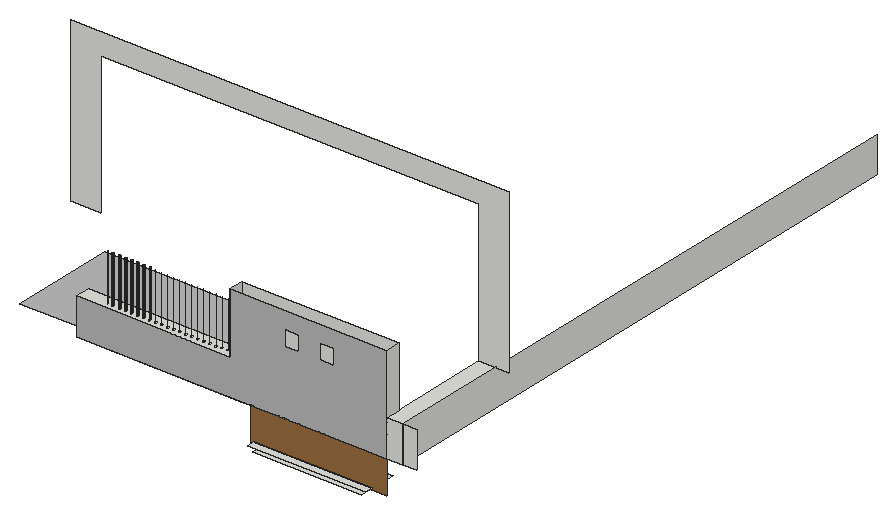
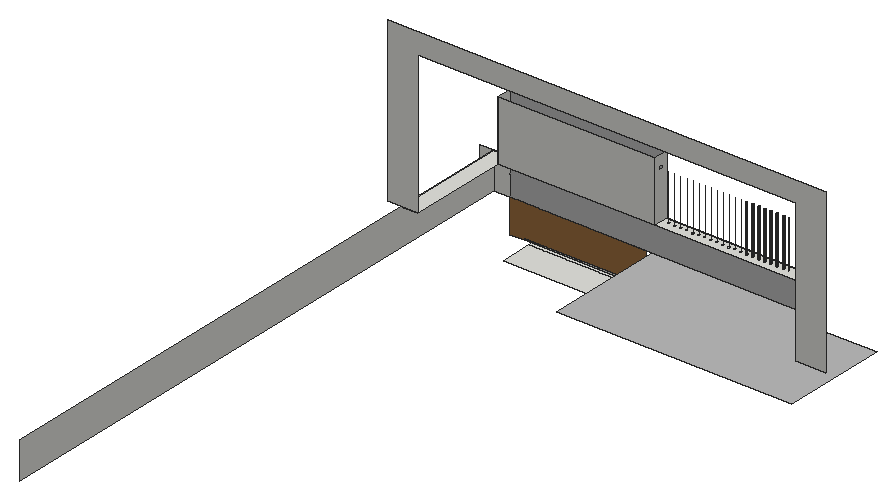
# SketchUp Ruby script. Lengths in inches.
U = 1.inch
M = Sketchup.active_model
def pt(a) = Geom::Point3d.new(a.map { |v| v * U })
def face(e, loops, mat)
  f = e.add_face(loops[0].map { |a| pt(a) })
  loops[1..].each { |l| e.add_face(l.map { |a| pt(a) }).erase! }
  f.material = f.back_material = mat if mat
  f
end
# faces: each face lists its corners as indices into pts; further lists are holes
def faces(e, pts, list, mat = nil) = list.each { |f| face(e, (f[0].is_a?(Array) ? f : [f]).map { |l| l.map { |i| pts[i] } }, mat) }
# xy, xz, yz: faces in a plane at the given z, y or x. An outline is a flat list of corners, or four numbers for a rectangle; further outlines are holes
def ring(l) = l.size == 4 ? [[l[0], l[1]], [l[2], l[1]], [l[2], l[3]], [l[0], l[3]]] : l.each_slice(2).to_a
def flat(e, list, mat, &to3) = list.each { |f| face(e, (f[0].is_a?(Array) ? f : [f]).map { |l| ring(l).map { |u, v| to3.(u, v) } }, mat) }
def xy(e, z, list, mat = nil) = flat(e, list, mat) { |x, y| [x, y, z] }
def xz(e, y, list, mat = nil) = flat(e, list, mat) { |x, z| [x, y, z] }
def yz(e, x, list, mat = nil) = flat(e, list, mat) { |y, z| [x, y, z] }
def lines(e, pts, list) = list.each { |a, b| e.add_line(pt(pts[a]), pt(pts[b])) }
# prism: a flat outline (further loops are holes) pulled along v
def prism(e, loops, v, mat = nil)
  f = face(e, loops, mat); d = Geom::Vector3d.new(v.map { |x| x * U })
  f.pushpull(f.normal.samedirection?(d) ? d.length : -d.length)
end
def box(e, o, s, mat = nil) = prism(e, [[o, [o[0] + s[0], o[1], o[2]], [o[0] + s[0], o[1] + s[1], o[2]], [o[0], o[1] + s[1], o[2]]]], [0, 0, s[2]], mat)
def at(x, y, z, deg = 0) = Geom::Transformation.translation(pt([x, y, z])) * Geom::Transformation.rotation(ORIGIN, Z_AXIS, deg.degrees)
def axes(o, x, y, z) = Geom::Transformation.new([*x, 0, *y, 0, *z, 0, *pt(o).to_a, 1])
def part(name) = M.definitions.add(name)
# library, detail: a bought-in or finely detailed component or shape, given as its bounding box
def library(name, o, s) = part(name).tap { |d| box(d.entities, o, s) }
def detail(e, o, s) = box(e.add_group.entities, o, s)
def put(e, d, t, mat = nil) = e.add_instance(d, t).tap { |i| i.material = mat if mat }
def group(e, t, mat = nil) = e.add_group.tap { |g| g.transformation = t; g.material = mat if mat }.entities
root = M.entities
M.materials.add("Generic").color = [155, 110, 63]
M.materials.add("Generic\#2").color = [186, 186, 186]
xy(root,951.29,[[543.83,116.625,654.26,124.5],[540.39,124.5,654.26,156.8125]])
xy(root,955.48,[[538.69,116.625,658.46,124.5]])
xy(root,987.75,[[359.25,124.5,359.25,138.74,290.4375,138.74,290.4375,246,528.75,246,528.75,124.5]],"Generic\#2")
xy(root,1024.625,[[483.23,129.75,483.02,129.78,482.82,129.86,482.66,129.99,482.53,130.16,482.45,130.36,482.42,130.57,482.45,130.78,482.53,130.97,482.66,131.14,482.82,131.27,483.02,131.35,483.23,131.38,483.44,131.35,483.64,131.27,483.81,131.14,483.93,130.97,484.02,130.78,484.04,130.57,484.02,130.36,483.93,130.16,483.81,129.99,483.64,129.86,483.44,129.78]])
xy(root,1024.6875,[[[359.25,124.5,514.86,139.4375],[501.61,129.75,501.4,129.78,501.2,129.86,501.03,129.99,500.9,130.16,500.82,130.36,500.79,130.57,500.82,130.78,500.9,130.97,501.03,131.14,501.2,131.27,501.4,131.35,501.61,131.38,501.82,131.35,502.01,131.27,502.18,131.14,502.31,130.97,502.39,130.78,502.42,130.57,502.39,130.36,502.31,130.16,502.18,129.99,502.01,129.86,501.82,129.78],[495.61,129.75,495.4,129.78,495.2,129.86,495.03,129.99,494.9,130.16,494.82,130.36,494.79,130.57,494.82,130.78,494.9,130.97,495.03,131.14,495.2,131.27,495.4,131.35,495.61,131.38,495.82,131.35,496.01,131.27,496.18,131.14,496.31,130.97,496.39,130.78,496.42,130.57,496.39,130.36,496.31,130.16,496.18,129.99,496.01,129.86,495.82,129.78],[489.61,129.75,489.4,129.78,489.2,129.86,489.03,129.99,488.9,130.16,488.82,130.36,488.79,130.57,488.82,130.78,488.9,130.97,489.03,131.14,489.2,131.27,489.4,131.35,489.61,131.38,489.82,131.35,490.01,131.27,490.18,131.14,490.31,130.97,490.39,130.78,490.42,130.57,490.39,130.36,490.31,130.16,490.18,129.99,490.01,129.86,489.82,129.78],[483.23,129.75,483.02,129.78,482.82,129.86,482.66,129.99,482.53,130.16,482.45,130.36,482.42,130.57,482.45,130.78,482.53,130.97,482.66,131.14,482.82,131.27,483.02,131.35,483.23,131.38,483.44,131.35,483.64,131.27,483.81,131.14,483.93,130.97,484.02,130.78,484.04,130.57,484.02,130.36,483.93,130.16,483.81,129.99,483.64,129.86,483.44,129.78],[477.17,129.75,476.96,129.78,476.76,129.86,476.59,129.99,476.46,130.16,476.38,130.36,476.36,130.57,476.38,130.78,476.46,130.97,476.59,131.14,476.76,131.27,476.96,131.35,477.17,131.38,477.38,131.35,477.57,131.27,477.74,131.14,477.87,130.97,477.95,130.78,477.98,130.57,477.95,130.36,477.87,130.16,477.74,129.99,477.57,129.86,477.38,129.78],[471.17,129.75,470.96,129.78,470.76,129.86,470.59,129.99,470.46,130.16,470.38,130.36,470.36,130.57,470.38,130.78,470.46,130.97,470.59,131.14,470.76,131.27,470.96,131.35,471.17,131.38,471.38,131.35,471.57,131.27,471.74,131.14,471.87,130.97,471.95,130.78,471.98,130.57,471.95,130.36,471.87,130.16,471.74,129.99,471.57,129.86,471.38,129.78],[464.79,129.75,464.58,129.78,464.39,129.86,464.22,129.99,464.09,130.16,464.01,130.36,463.98,130.57,464.01,130.78,464.09,130.97,464.22,131.14,464.39,131.27,464.58,131.35,464.79,131.38,465,131.35,465.2,131.27,465.37,131.14,465.5,130.97,465.58,130.78,465.61,130.57,465.58,130.36,465.5,130.16,465.37,129.99,465.2,129.86,465,129.78],[458.54,129.75,458.33,129.78,458.14,129.86,457.97,129.99,457.84,130.16,457.76,130.36,457.73,130.57,457.76,130.78,457.84,130.97,457.97,131.14,458.14,131.27,458.33,131.35,458.54,131.38,458.75,131.35,458.95,131.27,459.12,131.14,459.25,130.97,459.33,130.78,459.36,130.57,459.33,130.36,459.25,130.16,459.12,129.99,458.95,129.86,458.75,129.78],[452.61,129.75,452.4,129.78,452.2,129.86,452.03,129.99,451.9,130.16,451.82,130.36,451.79,130.57,451.82,130.78,451.9,130.97,452.03,131.14,452.2,131.27,452.4,131.35,452.61,131.38,452.82,131.35,453.01,131.27,453.18,131.14,453.31,130.97,453.39,130.78,453.42,130.57,453.39,130.36,453.31,130.16,453.18,129.99,453.01,129.86,452.82,129.78],[446.36,129.75,446.15,129.78,445.95,129.86,445.78,129.99,445.65,130.16,445.57,130.36,445.54,130.57,445.57,130.78,445.65,130.97,445.78,131.14,445.95,131.27,446.15,131.35,446.36,131.38,446.57,131.35,446.76,131.27,446.93,131.14,447.06,130.97,447.14,130.78,447.17,130.57,447.14,130.36,447.06,130.16,446.93,129.99,446.76,129.86,446.57,129.78],[440.36,129.75,440.15,129.78,439.95,129.86,439.78,129.99,439.65,130.16,439.57,130.36,439.54,130.57,439.57,130.78,439.65,130.97,439.78,131.14,439.95,131.27,440.15,131.35,440.36,131.38,440.57,131.35,440.76,131.27,440.93,131.14,441.06,130.97,441.14,130.78,441.17,130.57,441.14,130.36,441.06,130.16,440.93,129.99,440.76,129.86,440.57,129.78],[434.23,129.75,434.02,129.78,433.82,129.86,433.66,129.99,433.53,130.16,433.45,130.36,433.42,130.57,433.45,130.78,433.53,130.97,433.66,131.14,433.82,131.27,434.02,131.35,434.23,131.38,434.44,131.35,434.64,131.27,434.81,131.14,434.93,130.97,435.02,130.78,435.04,130.57,435.02,130.36,434.93,130.16,434.81,129.99,434.64,129.86,434.44,129.78],[428.17,129.75,427.96,129.78,427.76,129.86,427.59,129.99,427.46,130.16,427.38,130.36,427.36,130.57,427.38,130.78,427.46,130.97,427.59,131.14,427.76,131.27,427.96,131.35,428.17,131.38,428.38,131.35,428.57,131.27,428.74,131.14,428.87,130.97,428.95,130.78,428.98,130.57,428.95,130.36,428.87,130.16,428.74,129.99,428.57,129.86,428.38,129.78],[421.98,129.75,421.77,129.78,421.57,129.86,421.41,129.99,421.28,130.16,421.2,130.36,421.17,130.57,421.2,130.78,421.28,130.97,421.41,131.14,421.57,131.27,421.77,131.35,421.98,131.38,422.19,131.35,422.39,131.27,422.56,131.14,422.68,130.97,422.77,130.78,422.79,130.57,422.77,130.36,422.68,130.16,422.56,129.99,422.39,129.86,422.19,129.78],[415.86,129.75,415.65,129.78,415.45,129.86,415.28,129.99,415.15,130.16,415.07,130.36,415.04,130.57,415.07,130.78,415.15,130.97,415.28,131.14,415.45,131.27,415.65,131.35,415.86,131.38,416.07,131.35,416.26,131.27,416.43,131.14,416.56,130.97,416.64,130.78,416.67,130.57,416.64,130.36,416.56,130.16,416.43,129.99,416.26,129.86,416.07,129.78],[409.73,129.75,409.52,129.78,409.32,129.86,409.16,129.99,409.03,130.16,408.95,130.36,408.92,130.57,408.95,130.78,409.03,130.97,409.16,131.14,409.32,131.27,409.52,131.35,409.73,131.38,409.94,131.35,410.14,131.27,410.31,131.14,410.43,130.97,410.52,130.78,410.54,130.57,410.52,130.36,410.43,130.16,410.31,129.99,410.14,129.86,409.94,129.78],[403.61,129.75,403.4,129.78,403.2,129.86,403.03,129.99,402.9,130.16,402.82,130.36,402.79,130.57,402.82,130.78,402.9,130.97,403.03,131.14,403.2,131.27,403.4,131.35,403.61,131.38,403.82,131.35,404.01,131.27,404.18,131.14,404.31,130.97,404.39,130.78,404.42,130.57,404.39,130.36,404.31,130.16,404.18,129.99,404.01,129.86,403.82,129.78],[397.54,129.75,397.33,129.78,397.14,129.86,396.97,129.99,396.84,130.16,396.76,130.36,396.73,130.57,396.76,130.78,396.84,130.97,396.97,131.14,397.14,131.27,397.33,131.35,397.54,131.38,397.75,131.35,397.95,131.27,398.12,131.14,398.25,130.97,398.33,130.78,398.36,130.57,398.33,130.36,398.25,130.16,398.12,129.99,397.95,129.86,397.75,129.78],[391.23,129.75,391.02,129.78,390.82,129.86,390.66,129.99,390.53,130.16,390.45,130.36,390.42,130.57,390.45,130.78,390.53,130.97,390.66,131.14,390.82,131.27,391.02,131.35,391.23,131.38,391.44,131.35,391.64,131.27,391.81,131.14,391.93,130.97,392.02,130.78,392.04,130.57,392.02,130.36,391.93,130.16,391.81,129.99,391.64,129.86,391.44,129.78],[385.23,129.75,385.02,129.78,384.82,129.86,384.66,129.99,384.53,130.16,384.45,130.36,384.42,130.57,384.45,130.78,384.53,130.97,384.66,131.14,384.82,131.27,385.02,131.35,385.23,131.38,385.44,131.35,385.64,131.27,385.81,131.14,385.93,130.97,386.02,130.78,386.04,130.57,386.02,130.36,385.93,130.16,385.81,129.99,385.64,129.86,385.44,129.78],[378.98,129.75,378.77,129.78,378.57,129.86,378.41,129.99,378.28,130.16,378.2,130.36,378.17,130.57,378.2,130.78,378.28,130.97,378.41,131.14,378.57,131.27,378.77,131.35,378.98,131.38,379.19,131.35,379.39,131.27,379.56,131.14,379.68,130.97,379.77,130.78,379.79,130.57,379.77,130.36,379.68,130.16,379.56,129.99,379.39,129.86,379.19,129.78],[372.73,129.75,372.52,129.78,372.32,129.86,372.16,129.99,372.03,130.16,371.95,130.36,371.92,130.57,371.95,130.78,372.03,130.97,372.16,131.14,372.32,131.27,372.52,131.35,372.73,131.38,372.94,131.35,373.14,131.27,373.31,131.14,373.43,130.97,373.52,130.78,373.54,130.57,373.52,130.36,373.43,130.16,373.31,129.99,373.14,129.86,372.94,129.78],[366.79,129.75,366.58,129.78,366.39,129.86,366.22,129.99,366.09,130.16,366.01,130.36,365.98,130.57,366.01,130.78,366.09,130.97,366.22,131.14,366.39,131.27,366.58,131.35,366.79,131.38,367,131.35,367.2,131.27,367.37,131.14,367.5,130.97,367.58,130.78,367.61,130.57,367.58,130.36,367.5,130.16,367.37,129.99,367.2,129.86,367,129.78],[360.79,129.75,360.58,129.78,360.39,129.86,360.22,129.99,360.09,130.16,360.01,130.36,359.98,130.57,360.01,130.78,360.09,130.97,360.22,131.14,360.39,131.27,360.58,131.35,360.79,131.38,361,131.35,361.2,131.27,361.37,131.14,361.5,130.97,361.58,130.78,361.61,130.57,361.58,130.36,361.5,130.16,361.37,129.99,361.2,129.86,361,129.78],[507.61,129.75,507.4,129.78,507.2,129.86,507.03,129.99,506.9,130.16,506.82,130.36,506.79,130.57,506.82,130.78,506.9,130.97,507.03,131.14,507.2,131.27,507.4,131.35,507.61,131.38,507.82,131.35,508.01,131.27,508.18,131.14,508.31,130.97,508.39,130.78,508.42,130.57,508.39,130.36,508.31,130.16,508.18,129.99,508.01,129.86,507.82,129.78]],[673.48,124.5,690.4375,241.25],[391.23,129.75,391.02,129.78,390.82,129.86,390.66,129.99,390.53,130.16,390.45,130.36,390.42,130.57,390.45,130.78,390.53,130.97,390.66,131.14,390.82,131.27,391.02,131.35,391.23,131.38,391.44,131.35,391.64,131.27,391.81,131.14,391.93,130.97,392.02,130.78,392.04,130.57,392.02,130.36,391.93,130.16,391.81,129.99,391.64,129.86,391.44,129.78],[397.54,129.75,397.33,129.78,397.14,129.86,396.97,129.99,396.84,130.16,396.76,130.36,396.73,130.57,396.76,130.78,396.84,130.97,396.97,131.14,397.14,131.27,397.33,131.35,397.54,131.38,397.75,131.35,397.95,131.27,398.12,131.14,398.25,130.97,398.33,130.78,398.36,130.57,398.33,130.36,398.25,130.16,398.12,129.99,397.95,129.86,397.75,129.78],[403.61,129.75,403.4,129.78,403.2,129.86,403.03,129.99,402.9,130.16,402.82,130.36,402.79,130.57,402.82,130.78,402.9,130.97,403.03,131.14,403.2,131.27,403.4,131.35,403.61,131.38,403.82,131.35,404.01,131.27,404.18,131.14,404.31,130.97,404.39,130.78,404.42,130.57,404.39,130.36,404.31,130.16,404.18,129.99,404.01,129.86,403.82,129.78],
  [409.73,129.75,409.52,129.78,409.32,129.86,409.16,129.99,409.03,130.16,408.95,130.36,408.92,130.57,408.95,130.78,409.03,130.97,409.16,131.14,409.32,131.27,409.52,131.35,409.73,131.38,409.94,131.35,410.14,131.27,410.31,131.14,410.43,130.97,410.52,130.78,410.54,130.57,410.52,130.36,410.43,130.16,410.31,129.99,410.14,129.86,409.94,129.78],[415.86,129.75,415.65,129.78,415.45,129.86,415.28,129.99,415.15,130.16,415.07,130.36,415.04,130.57,415.07,130.78,415.15,130.97,415.28,131.14,415.45,131.27,415.65,131.35,415.86,131.38,416.07,131.35,416.26,131.27,416.43,131.14,416.56,130.97,416.64,130.78,416.67,130.57,416.64,130.36,416.56,130.16,416.43,129.99,416.26,129.86,416.07,129.78],[421.98,129.75,421.77,129.78,421.57,129.86,421.41,129.99,421.28,130.16,421.2,130.36,421.17,130.57,421.2,130.78,421.28,130.97,421.41,131.14,421.57,131.27,421.77,131.35,421.98,131.38,422.19,131.35,422.39,131.27,422.56,131.14,422.68,130.97,422.77,130.78,422.79,130.57,422.77,130.36,422.68,130.16,422.56,129.99,422.39,129.86,422.19,129.78],[428.17,129.75,427.96,129.78,427.76,129.86,427.59,129.99,427.46,130.16,427.38,130.36,427.36,130.57,427.38,130.78,427.46,130.97,427.59,131.14,427.76,131.27,427.96,131.35,428.17,131.38,428.38,131.35,428.57,131.27,428.74,131.14,428.87,130.97,428.95,130.78,428.98,130.57,428.95,130.36,428.87,130.16,428.74,129.99,428.57,129.86,428.38,129.78],[434.23,129.75,434.02,129.78,433.82,129.86,433.66,129.99,433.53,130.16,433.45,130.36,433.42,130.57,433.45,130.78,433.53,130.97,433.66,131.14,433.82,131.27,434.02,131.35,434.23,131.38,434.44,131.35,434.64,131.27,434.81,131.14,434.93,130.97,435.02,130.78,435.04,130.57,435.02,130.36,434.93,130.16,434.81,129.99,434.64,129.86,434.44,129.78],
  [440.36,129.75,440.15,129.78,439.95,129.86,439.78,129.99,439.65,130.16,439.57,130.36,439.54,130.57,439.57,130.78,439.65,130.97,439.78,131.14,439.95,131.27,440.15,131.35,440.36,131.38,440.57,131.35,440.76,131.27,440.93,131.14,441.06,130.97,441.14,130.78,441.17,130.57,441.14,130.36,441.06,130.16,440.93,129.99,440.76,129.86,440.57,129.78],[446.36,129.75,446.15,129.78,445.95,129.86,445.78,129.99,445.65,130.16,445.57,130.36,445.54,130.57,445.57,130.78,445.65,130.97,445.78,131.14,445.95,131.27,446.15,131.35,446.36,131.38,446.57,131.35,446.76,131.27,446.93,131.14,447.06,130.97,447.14,130.78,447.17,130.57,447.14,130.36,447.06,130.16,446.93,129.99,446.76,129.86,446.57,129.78],[452.61,129.75,452.4,129.78,452.2,129.86,452.03,129.99,451.9,130.16,451.82,130.36,451.79,130.57,451.82,130.78,451.9,130.97,452.03,131.14,452.2,131.27,452.4,131.35,452.61,131.38,452.82,131.35,453.01,131.27,453.18,131.14,453.31,130.97,453.39,130.78,453.42,130.57,453.39,130.36,453.31,130.16,453.18,129.99,453.01,129.86,452.82,129.78],[458.54,129.75,458.33,129.78,458.14,129.86,457.97,129.99,457.84,130.16,457.76,130.36,457.73,130.57,457.76,130.78,457.84,130.97,457.97,131.14,458.14,131.27,458.33,131.35,458.54,131.38,458.75,131.35,458.95,131.27,459.12,131.14,459.25,130.97,459.33,130.78,459.36,130.57,459.33,130.36,459.25,130.16,459.12,129.99,458.95,129.86,458.75,129.78],[464.79,129.75,464.58,129.78,464.39,129.86,464.22,129.99,464.09,130.16,464.01,130.36,463.98,130.57,464.01,130.78,464.09,130.97,464.22,131.14,464.39,131.27,464.58,131.35,464.79,131.38,465,131.35,465.2,131.27,465.37,131.14,465.5,130.97,465.58,130.78,465.61,130.57,465.58,130.36,465.5,130.16,465.37,129.99,465.2,129.86,465,129.78],
  [471.17,129.75,470.96,129.78,470.76,129.86,470.59,129.99,470.46,130.16,470.38,130.36,470.36,130.57,470.38,130.78,470.46,130.97,470.59,131.14,470.76,131.27,470.96,131.35,471.17,131.38,471.38,131.35,471.57,131.27,471.74,131.14,471.87,130.97,471.95,130.78,471.98,130.57,471.95,130.36,471.87,130.16,471.74,129.99,471.57,129.86,471.38,129.78],[477.17,129.75,476.96,129.78,476.76,129.86,476.59,129.99,476.46,130.16,476.38,130.36,476.36,130.57,476.38,130.78,476.46,130.97,476.59,131.14,476.76,131.27,476.96,131.35,477.17,131.38,477.38,131.35,477.57,131.27,477.74,131.14,477.87,130.97,477.95,130.78,477.98,130.57,477.95,130.36,477.87,130.16,477.74,129.99,477.57,129.86,477.38,129.78],[483.23,129.75,483.02,129.78,482.82,129.86,482.66,129.99,482.53,130.16,482.45,130.36,482.42,130.57,482.45,130.78,482.53,130.97,482.66,131.14,482.82,131.27,483.02,131.35,483.23,131.38,483.44,131.35,483.64,131.27,483.81,131.14,483.93,130.97,484.02,130.78,484.04,130.57,484.02,130.36,483.93,130.16,483.81,129.99,483.64,129.86,483.44,129.78],[489.61,129.75,489.4,129.78,489.2,129.86,489.03,129.99,488.9,130.16,488.82,130.36,488.79,130.57,488.82,130.78,488.9,130.97,489.03,131.14,489.2,131.27,489.4,131.35,489.61,131.38,489.82,131.35,490.01,131.27,490.18,131.14,490.31,130.97,490.39,130.78,490.42,130.57,490.39,130.36,490.31,130.16,490.18,129.99,490.01,129.86,489.82,129.78],[495.61,129.75,495.4,129.78,495.2,129.86,495.03,129.99,494.9,130.16,494.82,130.36,494.79,130.57,494.82,130.78,494.9,130.97,495.03,131.14,495.2,131.27,495.4,131.35,495.61,131.38,495.82,131.35,496.01,131.27,496.18,131.14,496.31,130.97,496.39,130.78,496.42,130.57,496.39,130.36,496.31,130.16,496.18,129.99,496.01,129.86,495.82,129.78],
  [501.61,129.75,501.4,129.78,501.2,129.86,501.03,129.99,500.9,130.16,500.82,130.36,500.79,130.57,500.82,130.78,500.9,130.97,501.03,131.14,501.2,131.27,501.4,131.35,501.61,131.38,501.82,131.35,502.01,131.27,502.18,131.14,502.31,130.97,502.39,130.78,502.42,130.57,502.39,130.36,502.31,130.16,502.18,129.99,502.01,129.86,501.82,129.78],[507.61,129.75,507.4,129.78,507.2,129.86,507.03,129.99,506.9,130.16,506.82,130.36,506.79,130.57,506.82,130.78,506.9,130.97,507.03,131.14,507.2,131.27,507.4,131.35,507.61,131.38,507.82,131.35,508.01,131.27,508.18,131.14,508.31,130.97,508.39,130.78,508.42,130.57,508.39,130.36,508.31,130.16,508.18,129.99,508.01,129.86,507.82,129.78]])
xz(root,124.5,[[538.69,954,658.46,955.48],[673.48,987.75,690.4375,1024.6875],[690.4375,987.75,703.6875,1024.6875]])
xz(root,124.5,[[535.75,954,538.69,954,538.69,955.48,658.46,955.48,658.46,954,673.48,954,673.48,987.75,535.75,987.75]],"Generic")
xz(root,124.5,[[[359.25,987.75,673.48,987.75,673.48,1085.75,514.86,1085.75,514.86,1024.6875,359.25,1024.6875],[570.42,1053.3125,584.1,1069],[605.79,1053.3125,619.48,1069]]],"Generic\#2")
xz(root,139.4375,[[514.86,1024.6875,673.48,1085.75]])
xz(root,241.25,[[259.3125,1024.6875,259.3125,1189.3125,703.6875,1189.3125,703.6875,1024.6875,673.48,1024.6875,673.48,1168.125,290.4375,1168.125,290.4375,1024.6875]])
yz(root,514.86,[[[124.5,1024.6875,139.4375,1085.75],[128.48,1072.38,133.48,1075.32]]])
yz(root,673.48,[[124.5,1024.6875,139.4375,1085.75]])
yz(root,690.4375,[[124.5,987.75,724.5,1024.6875]])
p = [[483.02,129.78,1024.6875],[482.82,129.86,1024.6875],[482.82,129.86,1024.625],[483.02,129.78,1024.625],[483.23,129.75,1024.6875],[483.23,129.75,1024.625],
  [483.44,129.78,1024.6875],[483.44,129.78,1024.625],[483.64,129.86,1024.6875],[483.64,129.86,1024.625],[482.66,129.99,1024.6875],[482.66,129.99,1024.625],
  [483.81,129.99,1024.6875],[483.81,129.99,1024.625],[482.53,130.16,1024.6875],[482.53,130.16,1024.625],[483.93,130.16,1024.6875],[483.93,130.16,1024.625],
  [482.45,130.36,1024.6875],[482.45,130.36,1024.625],[484.02,130.36,1024.6875],[484.02,130.36,1024.625],[482.42,130.57,1024.6875],[482.42,130.57,1024.625],
  [484.04,130.57,1024.6875],[484.04,130.57,1024.625],[482.45,130.78,1024.6875],[482.45,130.78,1024.625],[484.02,130.78,1024.6875],[484.02,130.78,1024.625],
  [482.53,130.97,1024.6875],[482.53,130.97,1024.625],[483.93,130.97,1024.6875],[483.93,130.97,1024.625],[482.66,131.14,1024.6875],[482.66,131.14,1024.625],
  [483.81,131.14,1024.6875],[483.81,131.14,1024.625],[482.82,131.27,1024.6875],[482.82,131.27,1024.625],[483.64,131.27,1024.6875],[483.64,131.27,1024.625],
  [483.02,131.35,1024.6875],[483.02,131.35,1024.625],[483.44,131.35,1024.6875],[483.44,131.35,1024.625],[483.23,131.38,1024.6875],[483.23,131.38,1024.625],
  [390.82,129.86,1024.6875],[391.02,129.78,1024.6875],[391.02,129.78,1072.38],[390.82,129.86,1072.38],[391.23,129.75,1024.6875],[391.23,129.75,1072.38],
  [391.44,129.78,1024.6875],[391.44,129.78,1072.38],[391.64,129.86,1024.6875],[391.64,129.86,1072.38],[397.14,129.86,1024.6875],[397.33,129.78,1024.6875],
  [397.33,129.78,1072.38],[397.14,129.86,1072.38],[397.54,129.75,1024.6875],[397.54,129.75,1072.38],[397.75,129.78,1024.6875],[397.75,129.78,1072.38],
  [397.95,129.86,1024.6875],[397.95,129.86,1072.38],[403.2,129.86,1024.6875],[403.4,129.78,1024.6875],[403.4,129.78,1072.38],[403.2,129.86,1072.38],
  [403.61,129.75,1024.6875],[403.61,129.75,1072.38],[403.82,129.78,1024.6875],[403.82,129.78,1072.38],[404.01,129.86,1024.6875],[404.01,129.86,1072.38],
  [409.32,129.86,1024.6875],[409.52,129.78,1024.6875],[409.52,129.78,1072.38],[409.32,129.86,1072.38],[409.73,129.75,1024.6875],[409.73,129.75,1072.38],
  [409.94,129.78,1024.6875],[409.94,129.78,1072.38],[410.14,129.86,1024.6875],[410.14,129.86,1072.38],[415.45,129.86,1024.6875],[415.65,129.78,1024.6875],
  [415.65,129.78,1072.38],[415.45,129.86,1072.38],[415.86,129.75,1024.6875],[415.86,129.75,1072.38],[416.07,129.78,1024.6875],[416.07,129.78,1072.38],
  [416.26,129.86,1024.6875],[416.26,129.86,1072.38],[421.57,129.86,1024.6875],[421.77,129.78,1024.6875],[421.77,129.78,1072.38],[421.57,129.86,1072.38],
  [421.98,129.75,1024.6875],[421.98,129.75,1072.38],[422.19,129.78,1024.6875],[422.19,129.78,1072.38],[422.39,129.86,1024.6875],[422.39,129.86,1072.38],
  [390.66,129.99,1024.6875],[390.66,129.99,1072.38],[391.81,129.99,1024.6875],[391.81,129.99,1072.38],[396.97,129.99,1024.6875],[396.97,129.99,1072.38],
  [398.12,129.99,1024.6875],[398.12,129.99,1072.38],[403.03,129.99,1024.6875],[403.03,129.99,1072.38],[404.18,129.99,1024.6875],[404.18,129.99,1072.38],
  [409.16,129.99,1024.6875],[409.16,129.99,1072.38],[410.31,129.99,1024.6875],[410.31,129.99,1072.38],[415.28,129.99,1024.6875],[415.28,129.99,1072.38],
  [416.43,129.99,1024.6875],[416.43,129.99,1072.38],[421.41,129.99,1024.6875],[421.41,129.99,1072.38],[422.56,129.99,1024.6875],[422.56,129.99,1072.38],
  [428.57,129.86,1024.6875],[428.74,129.99,1024.6875],[428.74,129.99,1072.38],[428.57,129.86,1072.38],[390.53,130.16,1024.6875],[390.53,130.16,1072.38],
  [391.93,130.16,1024.6875],[391.93,130.16,1072.38],[396.84,130.16,1024.6875],[396.84,130.16,1072.38],[398.25,130.16,1024.6875],[398.25,130.16,1072.38],
  [402.9,130.16,1024.6875],[402.9,130.16,1072.38],[404.31,130.16,1024.6875],[404.31,130.16,1072.38],[409.03,130.16,1024.6875],[409.03,130.16,1072.38],
  [410.43,130.16,1024.6875],[410.43,130.16,1072.38],[415.15,130.16,1024.6875],[415.15,130.16,1072.38],[416.56,130.16,1024.6875],[416.56,130.16,1072.38],
  [421.28,130.16,1024.6875],[421.28,130.16,1072.38],[422.68,130.16,1024.6875],[422.68,130.16,1072.38],[428.87,130.16,1024.6875],[428.87,130.16,1072.38],
  [390.45,130.36,1024.6875],[390.45,130.36,1072.38],[392.02,130.36,1024.6875],[392.02,130.36,1072.38],[396.76,130.36,1024.6875],[396.76,130.36,1072.38],
  [398.33,130.36,1024.6875],[398.33,130.36,1072.38],[402.82,130.36,1024.6875],[402.82,130.36,1072.38],[404.39,130.36,1024.6875],[404.39,130.36,1072.38],
  [408.95,130.36,1024.6875],[408.95,130.36,1072.38],[410.52,130.36,1024.6875],[410.52,130.36,1072.38],[415.07,130.36,1024.6875],[415.07,130.36,1072.38],
  [416.64,130.36,1024.6875],[416.64,130.36,1072.38],[421.2,130.36,1024.6875],[421.2,130.36,1072.38],[422.77,130.36,1024.6875],[422.77,130.36,1072.38],
  [428.95,130.36,1024.6875],[428.95,130.36,1072.38],[390.42,130.57,1024.6875],[390.42,130.57,1072.38],[392.04,130.57,1024.6875],[392.04,130.57,1072.38],
  [396.73,130.57,1024.6875],[396.73,130.57,1072.38],[398.36,130.57,1024.6875],[398.36,130.57,1072.38],[402.79,130.57,1024.6875],[402.79,130.57,1072.38],
  [404.42,130.57,1024.6875],[404.42,130.57,1072.38],[408.92,130.57,1024.6875],[408.92,130.57,1072.38],[410.54,130.57,1024.6875],[410.54,130.57,1072.38],
  [415.04,130.57,1024.6875],[415.04,130.57,1072.38],[416.67,130.57,1024.6875],[416.67,130.57,1072.38],[421.17,130.57,1024.6875],[421.17,130.57,1072.38],
  [422.79,130.57,1024.6875],[422.79,130.57,1072.38],[428.98,130.57,1024.6875],[428.98,130.57,1072.38],[386.04,130.57,1024.6875],[386.02,130.78,1024.6875],
  [386.02,130.78,1072.38],[386.04,130.57,1072.38],[390.45,130.78,1024.6875],[390.45,130.78,1072.38],[392.02,130.78,1024.6875],[392.02,130.78,1072.38],
  [396.76,130.78,1024.6875],[396.76,130.78,1072.38],[398.33,130.78,1024.6875],[398.33,130.78,1072.38],[402.82,130.78,1024.6875],[402.82,130.78,1072.38],
  [404.39,130.78,1024.6875],[404.39,130.78,1072.38],[408.95,130.78,1024.6875],[408.95,130.78,1072.38],[410.52,130.78,1024.6875],[410.52,130.78,1072.38],
  [415.07,130.78,1024.6875],[415.07,130.78,1072.38],[416.64,130.78,1024.6875],[416.64,130.78,1072.38],[421.2,130.78,1024.6875],[421.2,130.78,1072.38],
  [422.77,130.78,1024.6875],[422.77,130.78,1072.38],[428.95,130.78,1024.6875],[428.95,130.78,1072.38],[390.53,130.97,1024.6875],[390.53,130.97,1072.38],
  [391.93,130.97,1024.6875],[391.93,130.97,1072.38],[396.84,130.97,1024.6875],[396.84,130.97,1072.38],[398.25,130.97,1024.6875],[398.25,130.97,1072.38],
  [402.9,130.97,1024.6875],[402.9,130.97,1072.38],[404.31,130.97,1024.6875],[404.31,130.97,1072.38],[409.03,130.97,1024.6875],[409.03,130.97,1072.38],
  [410.43,130.97,1024.6875],[410.43,130.97,1072.38],[415.15,130.97,1024.6875],[415.15,130.97,1072.38],[416.56,130.97,1024.6875],[416.56,130.97,1072.38],
  [421.28,130.97,1024.6875],[421.28,130.97,1072.38],[422.68,130.97,1024.6875],[422.68,130.97,1072.38],[428.87,130.97,1024.6875],[428.87,130.97,1072.38],
  [390.66,131.14,1024.6875],[390.66,131.14,1072.38],[391.81,131.14,1024.6875],[391.81,131.14,1072.38],[396.97,131.14,1024.6875],[396.97,131.14,1072.38],
  [398.12,131.14,1024.6875],[398.12,131.14,1072.38],[403.03,131.14,1024.6875],[403.03,131.14,1072.38],[404.18,131.14,1024.6875],[404.18,131.14,1072.38],
  [409.16,131.14,1024.6875],[409.16,131.14,1072.38],[410.31,131.14,1024.6875],[410.31,131.14,1072.38],[415.28,131.14,1024.6875],[415.28,131.14,1072.38],
  [416.43,131.14,1024.6875],[416.43,131.14,1072.38],[421.41,131.14,1024.6875],[421.41,131.14,1072.38],[422.56,131.14,1024.6875],[422.56,131.14,1072.38],
  [428.74,131.14,1024.6875],[428.74,131.14,1072.38],[390.82,131.27,1024.6875],[390.82,131.27,1072.38],[391.64,131.27,1024.6875],[391.64,131.27,1072.38],
  [397.14,131.27,1024.6875],[397.14,131.27,1072.38],[397.95,131.27,1024.6875],[397.95,131.27,1072.38],[403.2,131.27,1024.6875],[403.2,131.27,1072.38],
  [404.01,131.27,1024.6875],[404.01,131.27,1072.38],[409.32,131.27,1024.6875],[409.32,131.27,1072.38],[410.14,131.27,1024.6875],[410.14,131.27,1072.38],
  [415.45,131.27,1024.6875],[415.45,131.27,1072.38],[416.26,131.27,1024.6875],[416.26,131.27,1072.38],[421.57,131.27,1024.6875],[421.57,131.27,1072.38],
  [422.39,131.27,1024.6875],[422.39,131.27,1072.38],[427.76,131.27,1024.6875],[427.59,131.14,1024.6875],[427.59,131.14,1072.38],[427.76,131.27,1072.38],
  [428.57,131.27,1024.6875],[428.57,131.27,1072.38],[391.02,131.35,1024.6875],[391.02,131.35,1072.38],[391.44,131.35,1024.6875],[391.44,131.35,1072.38],
  [397.33,131.35,1024.6875],[397.33,131.35,1072.38],[397.75,131.35,1024.6875],[397.75,131.35,1072.38],[403.4,131.35,1024.6875],[403.4,131.35,1072.38],
  [403.82,131.35,1024.6875],[403.82,131.35,1072.38],[409.52,131.35,1024.6875],[409.52,131.35,1072.38],[409.94,131.35,1024.6875],[409.94,131.35,1072.38],
  [415.65,131.35,1024.6875],[415.65,131.35,1072.38],[416.07,131.35,1024.6875],[416.07,131.35,1072.38],[421.77,131.35,1024.6875],[421.77,131.35,1072.38],
  [422.19,131.35,1024.6875],[422.19,131.35,1072.38],[427.96,131.35,1024.6875],[427.96,131.35,1072.38],[428.38,131.35,1024.6875],[428.38,131.35,1072.38],
  [391.23,131.38,1024.6875],[391.23,131.38,1072.38],[397.54,131.38,1024.6875],[397.54,131.38,1072.38],[403.61,131.38,1024.6875],[403.61,131.38,1072.38],
  [409.73,131.38,1024.6875],[409.73,131.38,1072.38],[415.86,131.38,1024.6875],[415.86,131.38,1072.38],[421.98,131.38,1024.6875],[421.98,131.38,1072.38],
  [428.17,131.38,1024.6875],[428.17,131.38,1072.38],[507.61,130.57,1072.38],[507.61,130.57,1024.6875],[501.48,130.57,1072.38],[501.48,130.57,1024.6875],
  [495.36,130.57,1072.38],[495.36,130.57,1024.6875],[489.23,130.57,1072.38],[489.23,130.57,1024.6875],[483.11,130.57,1072.38],[483.11,130.57,1024.6875],
  [476.98,130.57,1072.38],[476.98,130.57,1024.6875],[470.86,130.57,1072.38],[470.86,130.57,1024.6875],[464.73,130.57,1072.38],[464.73,130.57,1024.6875],
  [458.61,130.57,1072.38],[458.61,130.57,1024.6875],[452.48,130.57,1072.38],[452.48,130.57,1024.6875],[446.36,130.57,1072.38],[446.36,130.57,1024.6875],
  [440.23,130.57,1072.38],[440.23,130.57,1024.6875],[434.11,130.57,1072.38],[434.11,130.57,1024.6875],[427.98,130.57,1072.38],[427.98,130.57,1024.6875],
  [421.86,130.57,1072.38],[421.86,130.57,1024.6875],[415.73,130.57,1072.38],[415.73,130.57,1024.6875],[409.61,130.57,1072.38],[409.61,130.57,1024.6875],
  [403.48,130.57,1072.38],[403.48,130.57,1024.6875],[397.36,130.57,1072.38],[397.36,130.57,1024.6875],[391.23,130.57,1072.38],[391.23,130.57,1024.6875]]
faces(root,p,[[0,1,2,3],[4,0,3,5],[6,4,5,7],[8,6,7,9],[1,10,11,2],[12,8,9,13],[10,14,15,11],[16,12,13,17],
  [14,18,19,15],[20,16,17,21],[18,22,23,19],[24,20,21,25],[22,26,27,23],[28,24,25,29],[26,30,31,27],[32,28,29,33],
  [30,34,35,31],[36,32,33,37],[34,38,39,35],[40,36,37,41],[38,42,43,39],[44,40,41,45],[42,46,47,43],[46,44,45,47]])
faces(root,p,[[48,49,50,51],[49,52,53,50],[52,54,55,53],[54,56,57,55],[58,59,60,61],[59,62,63,60],[62,64,65,63],[64,66,67,65],
  [68,69,70,71],[69,72,73,70],[72,74,75,73],[74,76,77,75],[78,79,80,81],[79,82,83,80],[82,84,85,83],[84,86,87,85],
  [88,89,90,91],[89,92,93,90],[92,94,95,93],[94,96,97,95],[98,99,100,101],[99,102,103,100],[102,104,105,103],[104,106,107,105],
  [108,48,51,109],[56,110,111,57],[112,58,61,113],[66,114,115,67],[116,68,71,117],[76,118,119,77],[120,78,81,121],[86,122,123,87],
  [124,88,91,125],[96,126,127,97],[128,98,101,129],[106,130,131,107],[132,133,134,135],[136,108,109,137],[110,138,139,111],[140,112,113,141],
  [114,142,143,115],[144,116,117,145],[118,146,147,119],[148,120,121,149],[122,150,151,123],[152,124,125,153],[126,154,155,127],[156,128,129,157],
  [130,158,159,131],[133,160,161,134],[162,136,137,163],[138,164,165,139],[166,140,141,167],[142,168,169,143],[170,144,145,171],[146,172,173,147],
  [174,148,149,175],[150,176,177,151],[178,152,153,179],[154,180,181,155],[182,156,157,183],[158,184,185,159],[160,186,187,161],[188,162,163,189],
  [164,190,191,165],[192,166,167,193],[168,194,195,169],[196,170,171,197],[172,198,199,173],[200,174,175,201],[176,202,203,177],[204,178,179,205],
  [180,206,207,181],[208,182,183,209],[184,210,211,185],[186,212,213,187],[214,215,216,217],[218,188,189,219],[190,220,221,191],[222,192,193,223],
  [194,224,225,195],[226,196,197,227],[198,228,229,199],[230,200,201,231],[202,232,233,203],[234,204,205,235],[206,236,237,207],[238,208,209,239],
  [210,240,241,211],[212,242,243,213],[244,218,219,245],[220,246,247,221],[248,222,223,249],[224,250,251,225],[252,226,227,253],[228,254,255,229],
  [256,230,231,257],[232,258,259,233],[260,234,235,261],[236,262,263,237],[264,238,239,265],[240,266,267,241],[242,268,269,243],[270,244,245,271],
  [246,272,273,247],[274,248,249,275],[250,276,277,251],[278,252,253,279],[254,280,281,255],[282,256,257,283],[258,284,285,259],[286,260,261,287],
  [262,288,289,263],[290,264,265,291],[266,292,293,267],[268,294,295,269],[296,270,271,297],[272,298,299,273],[300,274,275,301],[276,302,303,277],
  [304,278,279,305],[280,306,307,281],[308,282,283,309],[284,310,311,285],[312,286,287,313],[288,314,315,289],[316,290,291,317],[292,318,319,293],
  [320,321,322,323],[294,324,325,295],[326,296,297,327],[298,328,329,299],[330,300,301,331],[302,332,333,303],[334,304,305,335],[306,336,337,307],
  [338,308,309,339],[310,340,341,311],[342,312,313,343],[314,344,345,315],[346,316,317,347],[318,348,349,319],[350,320,323,351],[324,352,353,325],
  [354,326,327,355],[328,354,355,329],[356,330,331,357],[332,356,357,333],[358,334,335,359],[336,358,359,337],[360,338,339,361],[340,360,361,341],
  [362,342,343,363],[344,362,363,345],[364,346,347,365],[348,364,365,349],[366,350,351,367],[352,366,367,353]],"Generic\#2")
lines(root,p,[[368,369],[370,371],[372,373],[374,375],[376,377],[378,379],[380,381],[382,383],[384,385],[386,387],[388,389],[390,391],
  [392,393],[394,395],[396,397],[398,399],[400,401],[402,403],[404,405],[406,407]])
